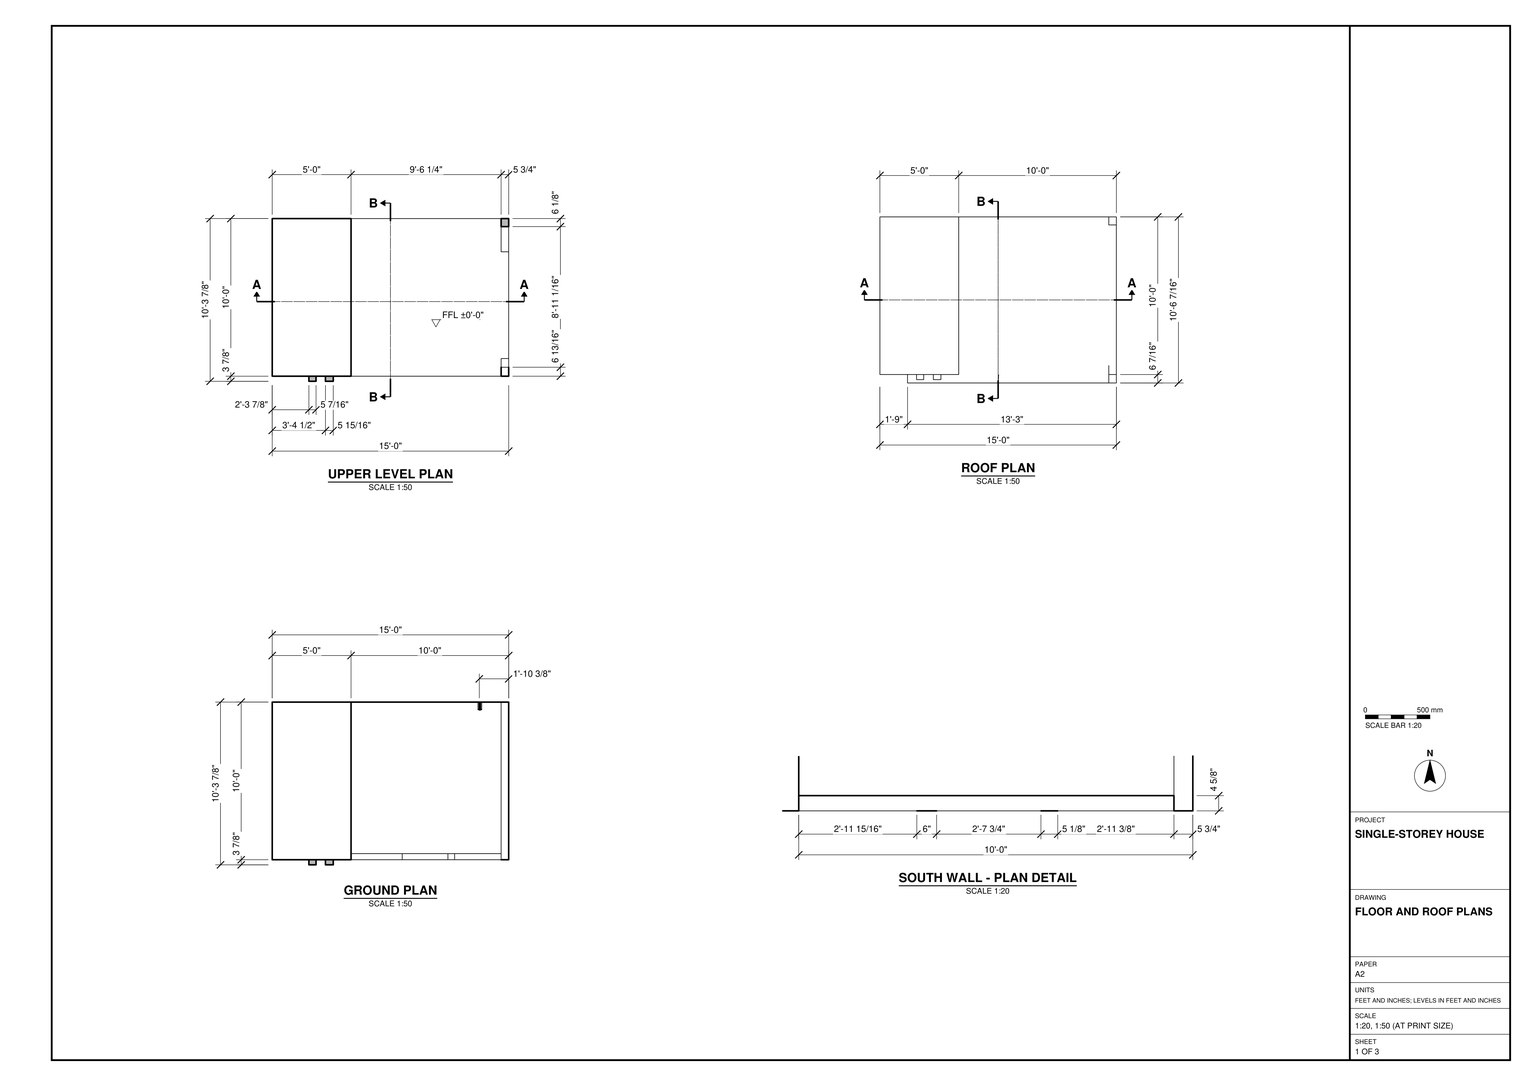
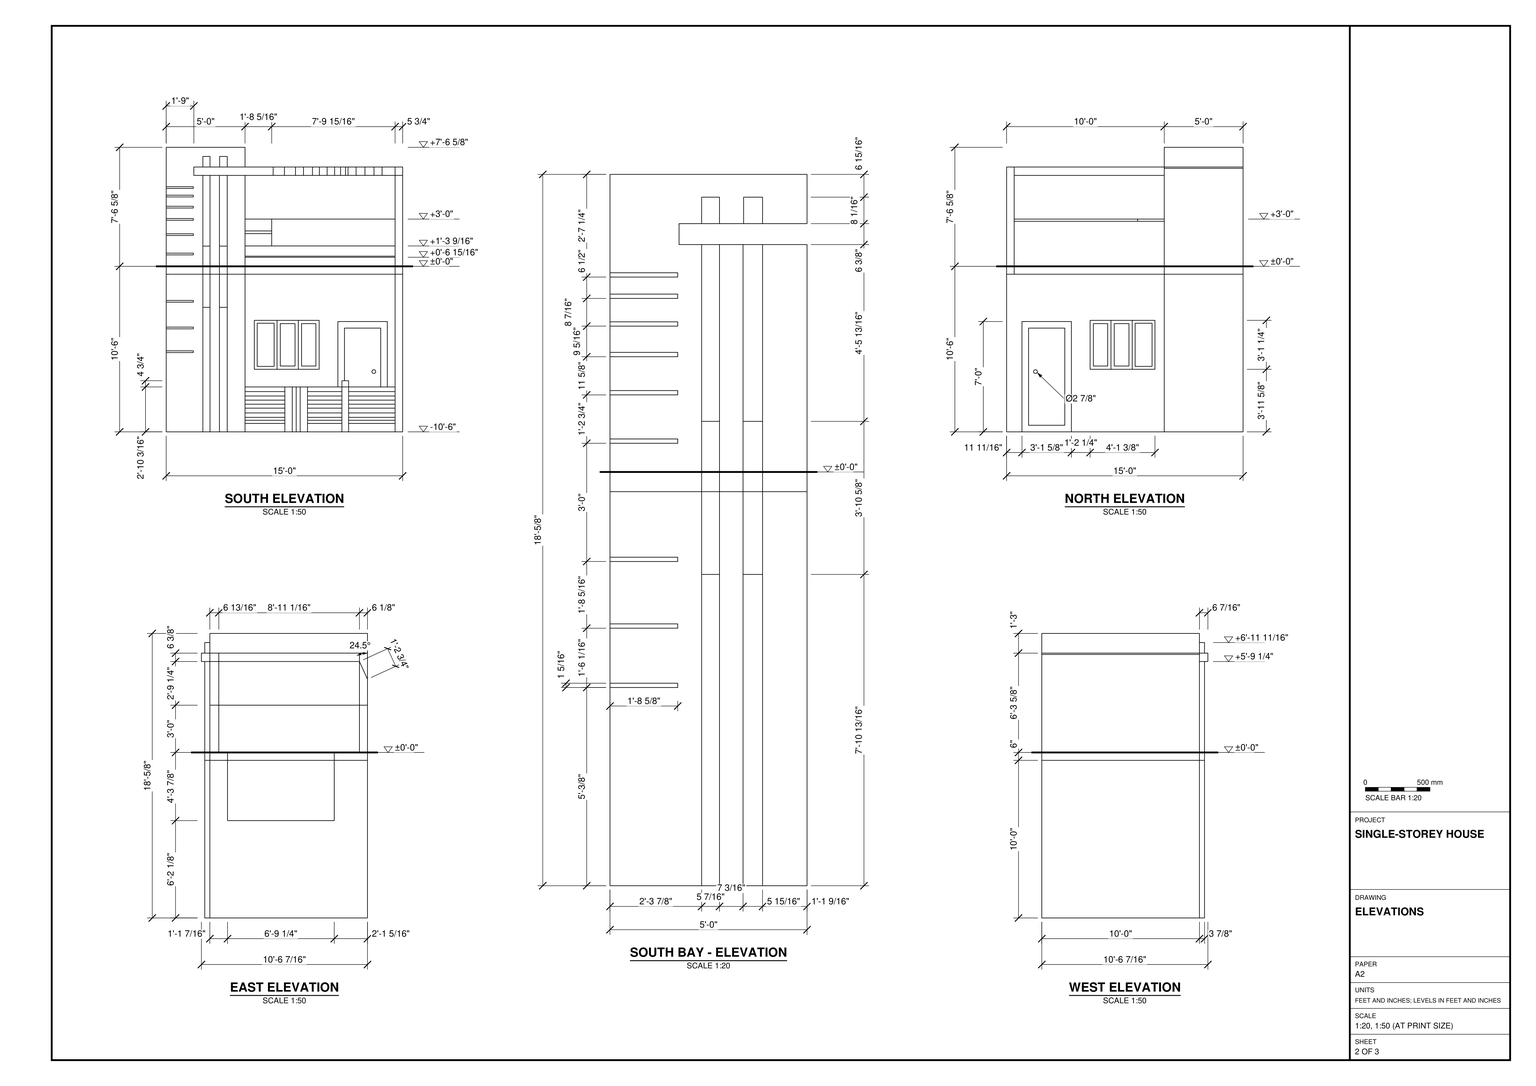
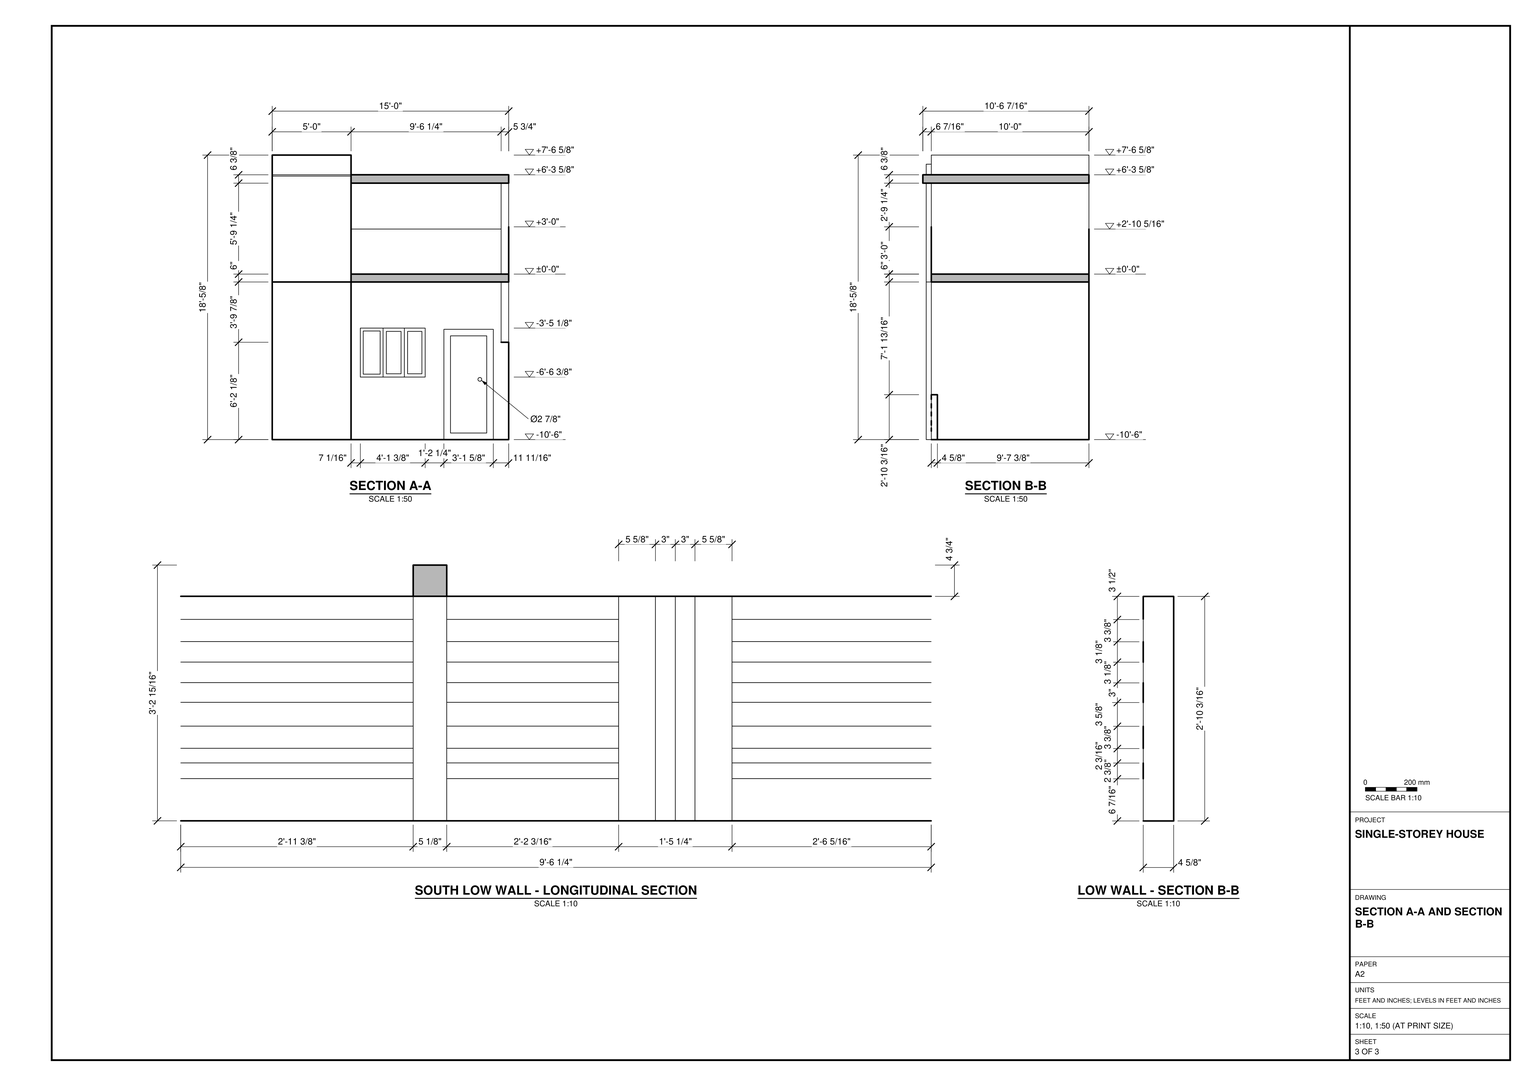
Build the house in SketchUp from task_files/diagram_01.pdf. Work in feet and inches. The overall dimensions, including the projections, are 15'-0" wide, 10'-6 7/16" deep and 18'-5/8" high. Use the finished floor marked ±0'-0" on the upper level plan as the datum. The base is at -10'-6", and the top of the taller bay is at +7'-6 5/8".

Lay out the 5'-0" west bay beside the 10'-0" east bay. Use sections A-A and B-B to place the slab and flat roof in the wider bay, and follow the roof plan for the projecting south edge. Model the walls at their drawn thicknesses. Fit the framed door and three-light window in the positions shown on the north elevation. On the south face of the taller bay, include the paired vertical strips and the short horizontal bands beside them. Use the enlarged low-wall details to model the banding and uprights across the lower part of the wider bay.

Keep walls, slabs, roof elements and any joinery or furniture pieces in separate groups or components, and use components for repeated parts. Any decor or loose items shown may be represented by suitable library components. Save one SketchUp model as output_files/single_storey_house_with_a_stepped_roofline.skp.

# SketchUp Ruby script. Lengths in inches.
U = 1.inch
M = Sketchup.active_model
def pt(a) = Geom::Point3d.new(a.map { |v| v * U })
def face(e, loops, mat)
  f = e.add_face(loops[0].map { |a| pt(a) })
  loops[1..].each { |l| e.add_face(l.map { |a| pt(a) }).erase! }
  f.material = f.back_material = mat if mat
  f
end
# faces: each face lists its corners as indices into pts; further lists are holes
def faces(e, pts, list, mat = nil) = list.each { |f| face(e, (f[0].is_a?(Array) ? f : [f]).map { |l| l.map { |i| pts[i] } }, mat) }
# xy, xz, yz: faces in a plane at the given z, y or x. An outline is a flat list of corners, or four numbers for a rectangle; further outlines are holes
def ring(l) = l.size == 4 ? [[l[0], l[1]], [l[2], l[1]], [l[2], l[3]], [l[0], l[3]]] : l.each_slice(2).to_a
def flat(e, list, mat, &to3) = list.each { |f| face(e, (f[0].is_a?(Array) ? f : [f]).map { |l| ring(l).map { |u, v| to3.(u, v) } }, mat) }
def xy(e, z, list, mat = nil) = flat(e, list, mat) { |x, y| [x, y, z] }
def xz(e, y, list, mat = nil) = flat(e, list, mat) { |x, z| [x, y, z] }
def yz(e, x, list, mat = nil) = flat(e, list, mat) { |y, z| [x, y, z] }
def lines(e, pts, list) = list.each { |a, b| e.add_line(pt(pts[a]), pt(pts[b])) }
# prism: a flat outline (further loops are holes) pulled along v
def prism(e, loops, v, mat = nil)
  f = face(e, loops, mat); d = Geom::Vector3d.new(v.map { |x| x * U })
  f.pushpull(f.normal.samedirection?(d) ? d.length : -d.length)
end
def box(e, o, s, mat = nil) = prism(e, [[o, [o[0] + s[0], o[1], o[2]], [o[0] + s[0], o[1] + s[1], o[2]], [o[0], o[1] + s[1], o[2]]]], [0, 0, s[2]], mat)
def at(x, y, z, deg = 0) = Geom::Transformation.translation(pt([x, y, z])) * Geom::Transformation.rotation(ORIGIN, Z_AXIS, deg.degrees)
def axes(o, x, y, z) = Geom::Transformation.new([*x, 0, *y, 0, *z, 0, *pt(o).to_a, 1])
def part(name) = M.definitions.add(name)
# library, detail: a bought-in or finely detailed component or shape, given as its bounding box
def library(name, o, s) = part(name).tap { |d| box(d.entities, o, s) }
def detail(e, o, s) = box(e.add_group.entities, o, s)
def put(e, d, t, mat = nil) = e.add_instance(d, t).tap { |i| i.material = mat if mat }
def group(e, t, mat = nil) = e.add_group.tap { |g| g.transformation = t; g.material = mat if mat }.entities
root = M.entities
M.materials.add("[0005_LightPink]").color = [255, 182, 193]
M.materials.add("[0010_Snow]").color = [255, 250, 250]
M.materials.add("[0018_Brown]").color = [165, 42, 42]
M.materials.add("[0022_Maroon]").color = [128, 0, 0]
M.materials.add("[0043_SaddleBrown]").color = [139, 69, 19]
M.materials.add("[0110_LightSlateGray]").color = [119, 136, 153]
M.materials.add("[0117_GhostWhite]").color = [248, 248, 255]
M.materials.add("[Carrera Marble]").color = [207, 207, 207]
M.materials.add("[Metal Rusted]").color = [184, 117, 91]
M.materials.add("[Translucent Glass Sky Reflection]").color = [126, 138, 183]
M.materials["[Translucent Glass Sky Reflection]"].alpha = 0.52
M.materials.add("[Translucent Glass Tinted]").color = [8, 201, 241]
M.materials["[Translucent Glass Tinted]"].alpha = 0.48
M.materials.add("[Wood Floor]").color = [155, 105, 61]
M.materials.add("[Wood Veneer 01]").color = [120, 70, 37]
xy(root,0,[[27.9,2.5625,33.34,6.4375],[40.51,2.5625,46.46,6.4375],[0,6.4375,60,126.4375],[60,6.4375,174.25,11.07],[174.25,6.4375,180,126.4375],
  [60,11.07,174.25,126.4375]])
xy(root,34.1875,[[133.75,6.4375,138.86,11.07]])
xy(root,34.1875,[[60,6.4375,98.95,11.07],[98.95,6.4375,133.75,11.07],[138.86,6.4375,174.25,11.07]],"[Metal Rusted]")
xy(root,38.9375,[[133.75,6.4375,138.86,11.07]],"[0010_Snow]")
xy(root,74.125,[[174.25,19.89,180,101.14]],"[0005_LightPink]")
xy(root,120,[[27.9,2.5625,33.34,6.4375],[40.51,2.5625,46.46,6.4375],[0,6.4375,60,126.4375]])
xy(root,120,[[174.25,6.4375,180,19.89],[174.25,101.14,180,126.4375]],"[0005_LightPink]")
xy(root,126,[[174.25,6.4375,180,13.25],[174.25,120.3125,180,126.4375]])
xy(root,195.25,[[21.03,0,21.03,6.4375,27.9,6.4375,27.9,2.5625,33.34,2.5625,33.34,6.4375,40.51,6.4375,40.51,2.5625,46.46,2.5625,46.46,6.4375,60,6.4375,60,0],[60,0,60,126.4375,174.25,126.4375,174.25,120.3125,180,120.3125,180,6.4375,174.25,6.4375,174.25,0],[174.25,0,180,6.4375],[27.9,2.5625,33.34,6.4375],[40.51,2.5625,46.46,6.4375]])
xy(root,201.625,[[21.03,0,174.25,0,174.25,6.4375,180,6.4375,180,120.3125,174.25,120.3125,174.25,126.4375,60,126.4375,60,6.4375,46.46,6.4375,46.46,2.5625,40.68,2.5625,40.68,6.4375,33.34,6.4375,33.34,2.5625,27.9,2.5625,27.9,6.4375,21.03,6.4375],[174.25,0,180,6.4375],[27.9,2.5625,33.34,6.4375],[40.68,2.5625,46.46,6.4375],[174.25,120.3125,180,126.4375]])
xy(root,209.6875,[[27.9,2.5625,33.34,6.4375],[40.68,2.5625,46.46,6.4375]],"[Carrera Marble]")
xy(root,216.625,[[0,6.4375,60,126.4375]])
xz(root,0,[[21.03,195.25,81.42,201.625],[89.98,195.25,98.41,201.625],[104.51,195.25,111.31,201.625],[116.59,195.25,122.51,201.625],[128.22,195.25,132.72,201.625],
  [138.41,195.25,144.55,201.625],[151.3,195.25,158.18,201.625],[164.34,195.25,174.25,201.625],[174.25,195.25,180,201.625]])
xz(root,0,[[81.42,195.25,89.98,201.625],[98.41,195.25,104.51,201.625],[111.31,195.25,116.59,201.625],[122.51,195.25,128.22,201.625],[132.72,195.25,136.48,201.625],
  [136.48,195.25,138.41,201.625],[144.55,195.25,151.3,201.625],[158.18,195.25,164.34,201.625]],"[0022_Maroon]")
xz(root,2.5625,[[27.9,94.8,33.34,120],[40.51,94.8,46.46,120],[27.9,120,33.34,141.42],[40.51,120,46.46,141.42]],"[0018_Brown]")
xz(root,2.5625,[[27.9,0,33.34,94.8],[40.51,0,46.46,94.8],[27.9,141.42,33.34,195.25],[40.51,141.42,46.46,195.25],[27.9,201.625,33.34,209.6875],
  [40.68,201.625,46.46,209.6875]],"[Carrera Marble]")
xz(root,6.4375,[[27.9,0,33.34,120],[33.34,0,40.51,120],[40.51,0,46.46,120],[46.46,0,60,120],[133.75,34.1875,138.86,38.9375],
  [0,60.36,20.625,61.68],[0,78.43,20.625,79.74],[0,98.74,20.625,100.05],[27.9,120,33.34,195.25],[33.34,120,40.51,195.25],
  [40.51,120,46.46,195.25],[46.46,120,60,195.25],[0,134.74,20.625,136.05],[0,149.48,20.625,150.79],[0,161.1,20.625,162.41],
  [0,170.41,20.625,171.73],[0,178.85,20.625,180.16],[0,185.35,20.625,186.66],[21.03,195.25,60,201.625],[174.25,195.25,180,201.625],
  [27.9,201.625,33.34,209.6875],[40.68,201.625,46.46,209.6875]])
xz(root,6.4375,[[174.25,0,180,120],[174.25,126,180,195.25]],"[0005_LightPink]")
xz(root,6.4375,[[133.75,0,138.86,34.1875]],"[0010_Snow]")
xz(root,6.4375,[[60,132.94,174.25,133.77]],"[0043_SaddleBrown]")
xz(root,6.4375,[[0,0,27.9,0,27.9,120,0,120,0,100.05,20.625,100.05,20.625,98.74,0,98.74,0,79.74,20.625,79.74,20.625,78.43,0,78.43,0,61.68,20.625,61.68,20.625,60.36,0,60.36],[0,120,27.9,120,27.9,195.25,21.03,195.25,21.03,201.625,27.9,201.625,27.9,209.6875,33.34,209.6875,33.34,201.625,40.68,201.625,40.68,209.6875,46.46,209.6875,46.46,201.625,60,201.625,60,216.625,0,216.625,0,186.66,20.625,186.66,20.625,185.35,0,185.35,0,180.16,20.625,180.16,20.625,178.85,0,178.85,0,171.73,20.625,171.73,20.625,170.41,0,170.41,0,162.41,20.625,162.41,20.625,161.1,0,161.1,0,150.79,20.625,150.79,20.625,149.48,0,149.48,0,136.05,20.625,136.05,20.625,134.74,0,134.74],[60,141.54,80.3,150.93],[60,152.97,80.3,162]],"[0110_LightSlateGray]")
xz(root,6.4375,[[60,126,174.25,132.94],[60,133.77,174.25,141.54],[60,150.93,80.3,152.97]],"[0117_GhostWhite]")
xz(root,6.4375,[[95.96,0,98.95,34.1875],[98.95,0,101.98,34.1875],[60,6.43,90.32,8.82],[107.58,6.43,133.75,8.82],[138.86,6.43,174.25,8.82],
  [60,11.04,90.32,14.42],[107.58,11.04,133.75,14.42],[138.86,11.04,174.25,14.42],[60,18.04,90.32,21.04],[107.58,18.04,133.75,21.04],
  [138.86,18.04,174.25,21.04],[60,24.17,90.32,27.29],[107.58,24.17,133.75,27.29],[138.86,24.17,174.25,27.29],[60,30.67,90.32,34.1875],
  [107.58,30.67,133.75,34.1875],[138.86,30.67,174.25,34.1875]],"[Metal Rusted]")
xz(root,6.4375,[[80.3,141.54,174.25,162]],"[Translucent Glass Tinted]")
xz(root,11.07,[[60,0,133.75,34.1875],[133.75,0,138.86,34.1875],[138.86,0,174.25,34.1875],[133.75,34.1875,138.86,38.9375]])
xz(root,19.89,[[174.25,74.125,180,120]])
xz(root,19.89,[[174.25,120,180,126]],"[0005_LightPink]")
xz(root,101.14,[[174.25,120,180,126]])
xz(root,101.14,[[174.25,74.125,180,120]],"[0005_LightPink]")
xz(root,120.3125,[[174.25,126,180,195.25],[174.25,195.25,180,201.625]])
xz(root,120.5625,[[158.04,44.44,158.41,44.49,158.76,44.63,159.06,44.86,159.28,45.16,159.43,45.51,159.48,45.88,159.43,46.25,159.28,46.6,159.06,46.89,158.76,47.12,158.41,47.27,158.04,47.31,157.67,47.27,157.32,47.12,157.02,46.89,156.79,46.6,156.65,46.25,156.6,45.88,156.65,45.51,156.79,45.16,157.02,44.86,157.32,44.63,157.67,44.49]],"[Wood Floor]")
xz(root,121.0625,[[158.04,44.44,157.67,44.49,157.32,44.63,157.02,44.86,156.79,45.16,156.65,45.51,156.6,45.88,156.65,46.25,156.79,46.6,157.02,46.89,157.32,47.12,157.67,47.27,158.04,47.31,158.41,47.27,158.76,47.12,159.06,46.89,159.28,46.6,159.43,46.25,159.48,45.88,159.43,45.51,159.28,45.16,159.06,44.86,158.76,44.63,158.41,44.49]],"[Wood Floor]")
xz(root,126.4375,[[0,0,60,120],[[60,0,60,126,174.25,126,174.25,120,180,120,180,0,168.3125,0,168.3125,84,130.6875,84,130.6875,0],[67.0625,47.625,116.4375,84.9]],[0,120,60,200.625],[60,126,174.25,160.3125],[174.25,126,180,201.625],
  [60,195.25,174.25,201.625],[0,200.625,60,201.625],[0,201.625,60,216.625]])
xz(root,126.4375,[[69.27,49.83,82.17,82.69],[86.87,50.12,98.07,82.41],[103.05,50.12,113.95,82.41]],"[Translucent Glass Sky Reflection]")
xz(root,126.4375,[[[135.7,5.02,163.3,78.98],[158.04,44.44,158.41,44.49,158.76,44.63,159.06,44.86,159.28,45.16,159.43,45.51,159.48,45.88,159.43,46.25,159.28,46.6,159.06,46.89,158.76,47.12,158.41,47.27,158.04,47.31,157.67,47.27,157.32,47.12,157.02,46.89,156.79,46.6,156.65,46.25,156.6,45.88,156.65,45.51,156.79,45.16,157.02,44.86,157.32,44.63,157.67,44.49]],[158.04,44.44,157.67,44.49,157.32,44.63,157.02,44.86,156.79,45.16,156.65,45.51,156.6,45.88,156.65,46.25,156.79,46.6,157.02,46.89,157.32,47.12,157.67,47.27,158.04,47.31,158.41,47.27,158.76,47.12,159.06,46.89,159.28,46.6,159.43,46.25,159.48,45.88,159.43,45.51,159.28,45.16,159.06,44.86,158.76,44.63,158.41,44.49]],"[Wood Floor]")
xz(root,126.4375,[[[130.6875,0,168.3125,84],[135.7,5.02,163.3,78.98]],[[67.0625,47.625,84.375,84.9],[69.27,49.83,82.17,82.69]],[[84.375,47.625,100.5625,84.9],[86.87,50.12,98.07,82.41]],[[100.5625,47.625,116.4375,84.9],[103.05,50.12,113.95,82.41]]],"[Wood Veneer 01]")
yz(root,0,[[6.4375,0,126.4375,120],[6.4375,120,126.4375,200.625],[6.4375,200.625,126.4375,201.625],[6.4375,201.625,126.4375,216.625]])
yz(root,21.03,[[0,195.25,6.4375,201.625]])
yz(root,27.9,[[2.5625,0,6.4375,120],[2.5625,120,6.4375,195.25],[2.5625,201.625,6.4375,209.6875]],"[Carrera Marble]")
yz(root,33.34,[[2.5625,0,6.4375,120],[2.5625,120,6.4375,195.25],[2.5625,201.625,6.4375,209.6875]],"[Carrera Marble]")
yz(root,40.51,[[2.5625,0,6.4375,120],[2.5625,120,6.4375,195.25]],"[Carrera Marble]")
yz(root,40.68,[[2.5625,201.625,6.4375,209.6875]],"[Carrera Marble]")
yz(root,46.46,[[2.5625,0,6.4375,120],[2.5625,120,6.4375,195.25],[2.5625,201.625,6.4375,209.6875]],"[Carrera Marble]")
yz(root,60,[[11.07,0,126.4375,0,126.4375,120,6.4375,120,6.4375,34.1875,11.07,34.1875],[6.4375,0,11.07,34.1875],[6.4375,120,126.4375,126],[6.4375,126,126.4375,195.25],[6.4375,195.25,126.4375,200.625],
  [6.4375,200.625,126.4375,201.625],[6.4375,201.625,126.4375,216.625]])
yz(root,133.75,[[6.4375,34.1875,11.07,38.9375]])
yz(root,138.86,[[6.4375,34.1875,11.07,38.9375]],"[0010_Snow]")
yz(root,174.25,[[6.4375,0,11.07,34.1875],[6.4375,74.125,19.89,120],[6.4375,126,13.25,201.625],[120.3125,126,126.4375,195.25],[0,195.25,6.4375,201.625],
  [120.3125,195.25,126.4375,201.625]])
yz(root,174.25,[[6.4375,120,19.89,126],[101.14,120,126.4375,126]],"[0005_LightPink]")
yz(root,180,[[6.4375,162,13.25,195.25],[0,195.25,6.4375,201.625],[6.4375,195.25,13.25,201.625]])
yz(root,180,[[6.4375,0,126.4375,0,126.4375,120,101.14,120,101.14,74.125,19.89,74.125,19.89,120,6.4375,120],[19.89,120,101.14,126],[6.4375,126,13.25,162],[13.25,126,120.3125,162],[120.3125,126,126.4375,162],
  [120.3125,162,126.4375,162,126.4375,181.8125,120.3125,195.25],[126.4375,181.8125,126.4375,201.625,120.3125,201.625,120.3125,195.25],[13.25,195.25,120.3125,201.625]],"[0005_LightPink]")
p = [[158.04,120.5625,44.44],[157.67,120.5625,44.49],[157.67,121.0625,44.49],[158.04,121.0625,44.44],[158.41,120.5625,44.49],[158.41,121.0625,44.49],
  [157.67,126.4375,44.49],[158.04,126.4375,44.44],[158.41,126.4375,44.49],[157.32,120.5625,44.63],[157.32,121.0625,44.63],[158.76,120.5625,44.63],
  [158.76,121.0625,44.63],[157.32,126.4375,44.63],[158.76,126.4375,44.63],[157.02,120.5625,44.86],[157.02,121.0625,44.86],[159.06,120.5625,44.86],
  [159.06,121.0625,44.86],[157.02,126.4375,44.86],[159.06,126.4375,44.86],[156.79,120.5625,45.16],[156.79,121.0625,45.16],[159.28,120.5625,45.16],
  [159.28,121.0625,45.16],[156.79,126.4375,45.16],[159.28,126.4375,45.16],[156.65,120.5625,45.51],[156.65,121.0625,45.51],[159.43,120.5625,45.51],
  [159.43,121.0625,45.51],[156.65,126.4375,45.51],[159.43,126.4375,45.51],[156.6,120.5625,45.88],[156.6,121.0625,45.88],[159.48,120.5625,45.88],
  [159.48,121.0625,45.88],[156.6,126.4375,45.88],[159.48,126.4375,45.88],[156.65,120.5625,46.25],[156.65,121.0625,46.25],[159.43,120.5625,46.25],
  [159.43,121.0625,46.25],[156.65,126.4375,46.25],[159.43,126.4375,46.25],[156.79,120.5625,46.6],[156.79,121.0625,46.6],[159.28,120.5625,46.6],
  [159.28,121.0625,46.6],[156.79,126.4375,46.6],[159.28,126.4375,46.6],[157.02,120.5625,46.89],[157.02,121.0625,46.89],[159.06,120.5625,46.89],
  [159.06,121.0625,46.89],[157.02,126.4375,46.89],[159.06,126.4375,46.89],[157.32,120.5625,47.12],[157.32,121.0625,47.12],[158.76,120.5625,47.12],
  [158.76,121.0625,47.12],[157.32,126.4375,47.12],[158.76,126.4375,47.12],[157.67,120.5625,47.27],[157.67,121.0625,47.27],[158.41,120.5625,47.27],
  [158.41,121.0625,47.27],[157.67,126.4375,47.27],[158.41,126.4375,47.27],[158.04,120.5625,47.31],[158.04,121.0625,47.31],[158.04,126.4375,47.31],
  [60,6.4375,120],[174.25,6.4375,120],[89.98,0,201.625],[98.41,126.4375,195.25],[90.32,6.4375,0],[90.32,6.4375,6.43],
  [90.32,6.4375,27.29],[90.32,6.4375,30.67],[90.32,6.4375,8.82],[90.32,6.4375,11.04],[90.32,6.4375,14.42],[90.32,6.4375,18.04],
  [90.32,6.4375,21.04],[90.32,6.4375,24.17],[107.58,6.4375,0],[107.58,6.4375,6.43],[107.58,6.4375,8.82],[107.58,6.4375,11.04],
  [107.58,6.4375,14.42],[107.58,6.4375,18.04],[107.58,6.4375,27.29],[107.58,6.4375,30.67],[107.58,6.4375,21.04],[107.58,6.4375,24.17]]
faces(root,p,[[0,1,2,3],[4,0,3,5],[6,7,3,2],[7,8,5,3],[1,9,10,2],[11,4,5,12],[13,6,2,10],[8,14,12,5],
  [9,15,16,10],[17,11,12,18],[19,13,10,16],[14,20,18,12],[15,21,22,16],[23,17,18,24],[25,19,16,22],[20,26,24,18],
  [21,27,28,22],[29,23,24,30],[31,25,22,28],[26,32,30,24],[27,33,34,28],[35,29,30,36],[37,31,28,34],[32,38,36,30],
  [33,39,40,34],[41,35,36,42],[43,37,34,40],[38,44,42,36],[39,45,46,40],[47,41,42,48],[49,43,40,46],[44,50,48,42],
  [45,51,52,46],[53,47,48,54],[55,49,46,52],[50,56,54,48],[51,57,58,52],[59,53,54,60],[61,55,52,58],[56,62,60,54],
  [57,63,64,58],[65,59,60,66],[67,61,58,64],[62,68,66,60],[63,69,70,64],[69,65,66,70],[71,67,64,70],[68,71,70,66]],"[Wood Floor]")
lines(root,p,[[72,73],[74,75],[76,77],[78,79],[80,81],[82,83],[84,85],[86,87],[88,89],[90,91],[92,93],[94,95]])
g1 = group(root,at(60,6.4375,120))
box(g1,[0,0,0],[120,120,6])
